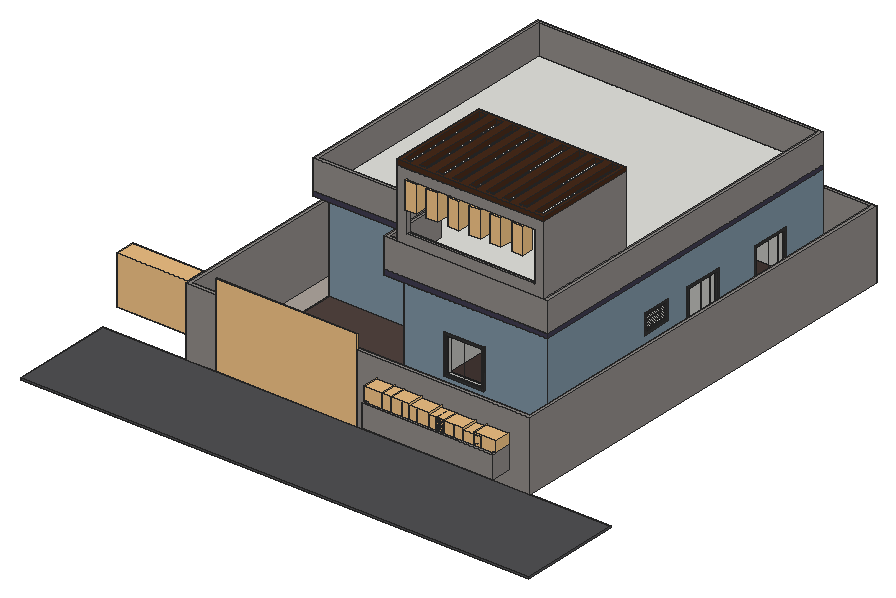
# SketchUp Ruby script. Lengths in inches.
U = 1.inch
M = Sketchup.active_model
def pt(a) = Geom::Point3d.new(a.map { |v| v * U })
def face(e, loops, mat)
  f = e.add_face(loops[0].map { |a| pt(a) })
  loops[1..].each { |l| e.add_face(l.map { |a| pt(a) }).erase! }
  f.material = f.back_material = mat if mat
  f
end
# faces: each face lists its corners as indices into pts; further lists are holes
def faces(e, pts, list, mat = nil) = list.each { |f| face(e, (f[0].is_a?(Array) ? f : [f]).map { |l| l.map { |i| pts[i] } }, mat) }
# xy, xz, yz: faces in a plane at the given z, y or x. An outline is a flat list of corners, or four numbers for a rectangle; further outlines are holes
def ring(l) = l.size == 4 ? [[l[0], l[1]], [l[2], l[1]], [l[2], l[3]], [l[0], l[3]]] : l.each_slice(2).to_a
def flat(e, list, mat, &to3) = list.each { |f| face(e, (f[0].is_a?(Array) ? f : [f]).map { |l| ring(l).map { |u, v| to3.(u, v) } }, mat) }
def xy(e, z, list, mat = nil) = flat(e, list, mat) { |x, y| [x, y, z] }
def xz(e, y, list, mat = nil) = flat(e, list, mat) { |x, z| [x, y, z] }
def yz(e, x, list, mat = nil) = flat(e, list, mat) { |y, z| [x, y, z] }
def lines(e, pts, list) = list.each { |a, b| e.add_line(pt(pts[a]), pt(pts[b])) }
# prism: a flat outline (further loops are holes) pulled along v
def prism(e, loops, v, mat = nil)
  f = face(e, loops, mat); d = Geom::Vector3d.new(v.map { |x| x * U })
  f.pushpull(f.normal.samedirection?(d) ? d.length : -d.length)
end
def box(e, o, s, mat = nil) = prism(e, [[o, [o[0] + s[0], o[1], o[2]], [o[0] + s[0], o[1] + s[1], o[2]], [o[0], o[1] + s[1], o[2]]]], [0, 0, s[2]], mat)
def at(x, y, z, deg = 0) = Geom::Transformation.translation(pt([x, y, z])) * Geom::Transformation.rotation(ORIGIN, Z_AXIS, deg.degrees)
def axes(o, x, y, z) = Geom::Transformation.new([*x, 0, *y, 0, *z, 0, *pt(o).to_a, 1])
def part(name) = M.definitions.add(name)
# library, detail: a bought-in or finely detailed component or shape, given as its bounding box
def library(name, o, s) = part(name).tap { |d| box(d.entities, o, s) }
def detail(e, o, s) = box(e.add_group.entities, o, s)
def put(e, d, t, mat = nil) = e.add_instance(d, t).tap { |i| i.material = mat if mat }
def group(e, t, mat = nil) = e.add_group.tap { |g| g.transformation = t; g.material = mat if mat }.entities
root = M.entities
M.materials.add("Asphalt A02 100cm").color = [81, 81, 83]
M.materials.add("Glass Green 001").color = [0, 0, 0]
M.materials["Glass Green 001"].alpha = 0.1
M.materials.add("Iron Blurry").color = [53, 53, 53]
M.materials.add("Marble Emperador Dark 150cm").color = [81, 67, 62]
M.materials.add("Tiles Simple H01 100cm").color = [173, 165, 157]
M.materials.add("Venetian Plaster Shadow 300cm").color = [61, 58, 77]
M.materials.add("Wall Paint Dusk Blue Semigloss 300cm").color = [122, 143, 157]
M.materials.add("Wall Paint Poised Taupe Semigloss 300cm").color = [140, 135, 132]
M.materials.add("Wenge Highgloss 300cm").color = [70, 42, 26]
c1 = library("gate 251k",[-0.18,0,0],[84.18,1.97,100.875])
c2 = library("Skimmia japonica Rubella 004",[-17.08,-16.64,-0.26],[33.2,34.59,28.81])
c3 = library("Hanging Plant 111-02",[-6.97,-7.06,-31.95],[13.94,14.12,31.95])
c4 = library("Dome Light",[-12,-12,0],[24,24,12])
c5 = part("Group\#31")
box(c5.entities,[0,0,0],[0.31,22,44])
c6 = part("Group\#33")
box(c6.entities,[0,0,0],[22,0.31,44])
c7 = part("Group\#35")
box(c7.entities,[0,0,0],[0.31,32,2])
c8 = part("Group\#37")
box(c8.entities,[-0.31,0,0],[0.31,22,44])
c9 = part("Group\#39")
box(c9.entities,[-0.31,0,0],[0.31,22,44])
c10 = part("Group\#41")
box(c10.entities,[0,0,0],[0.31,22,44])
c11 = part("Group\#43")
box(c11.entities,[0,0,0],[0.81,22,44])
c12 = part("Group\#45")
box(c12.entities,[0,0,0],[0.31,16,44])
put(root,c1,axes([309.25,125.79,8.27],[-2.04321,0,0],[0,1,0],[0,0,1]))
put(root,c2,axes([351.27,123.2,31.01],[1,0,0],[0,1,0],[0,0,1.35]))
put(root,c2,axes([373.16,123.2,31],[1,0,0],[0,1,0],[0,0,1.34812]))
put(root,c2,axes([397.15,123.2,30.99],[1,0,0],[0,1,0],[0,0,1.29341]))
put(root,c2,axes([415.51,123.2,30.98],[1,0,0],[0,1,0],[0,0,1.24092]))
put(root,c2,axes([439.16,123.2,30.97],[1,0,0],[0,1,0],[0,0,1.23466]))
put(root,c2,axes([461.16,123.2,30.96],[1,0,0],[0,1,0],[0,0,1.17781]))
put(root,c2,axes([482.18,123.2,30.98],[0.80733,0,0],[0,1,0],[0,0,1.24301]))
put(root,c3,at(320.25,202.29,248.27))
put(root,c3,at(345.8,202.29,248.27))
put(root,c3,at(372.54,202.29,248.27))
put(root,c3,at(398.6,202.29,248.27))
put(root,c3,at(423.8,202.29,248.27))
put(root,c3,at(450.02,202.29,248.27))
put(root,c4,axes([12.81,197.79,-6.4],[3.6267,0,0],[0,1,0],[0,0,4.8972]))
g1 = group(root,at(137.625,197.79,14.27))
xy(g1,0,[[0,0,172,0,172,101,136.6875,101,136.6875,105.5,172,105.5,172,138,181,138,181,9,339,9,339,133.5,217,133.5,217,196.5,227.5,196.5,227.5,192,221.5,192,221.5,138,264.5,138,264.5,143.4375,269,143.4375,269,138,339,138,339,192,269,192,269,179.4375,264.5,179.4375,264.5,192,263.5,192,263.5,196.5,339,196.5,339,274.5,224.5,274.5,224.5,279,339,279,339,411,176.5,411,176.5,279,188.5,279,188.5,274.5,160,274.5,160,279,172,279,172,411,9,411,9,279,124,279,124,274.5,85.5,274.5,85.5,202.5,81,202.5,81,274.5,9,274.5,9,154.5,81,154.5,81,166.5,85.5,166.5,85.5,150,9,150,9,105.5,81,105.5,81,114,85.5,114,85.5,105.5,100.6875,105.5,100.6875,101,0,101]],"Marble Emperador Dark 150cm")
xy(g1,36,[[222.5625,0,270.5625,9],[172,29.875,181,77.875],[0,110.375,9,146.375],[0,193.375,9,241.375],[339,210.875,348,258.875],
  [339,313.625,348,361.625],[0,327.125,9,375.125]])
xy(g1,60,[[339,145.8125,348,181.8125]])
xy(g1,84,[[222.5625,0,270.5625,9],[172,29.875,181,77.875],[100.6875,101,136.6875,105.5],[0,110.375,9,146.375],[81,114,85.5,150],
  [181,133.5,217,138],[264.5,143.4375,269,179.4375],[339,145.8125,348,181.8125],[81,166.5,85.5,202.5],[227.5,192,263.5,196.5],
  [0,193.375,9,241.375],[339,210.875,348,258.875],[124,274.5,160,279],[188.5,274.5,224.5,279],[339,313.625,348,361.625],
  [0,327.125,9,375.125]])
xy(g1,120,[[[172,0,348,0,348,420,0,420,0,101,172,101],[85.5,105.5,85.5,274.5,339,274.5,339,196.5,217,196.5,217,138,172,138,172,105.5],[9,279,172,411],[176.5,279,339,411],[181,9,339,133.5],[9,154.5,81,274.5],[269,138,339,192],[9,105.5,81,150],[221.5,138,264.5,192]]])
xz(g1,0,[[[172,0,348,120],[222.5625,36,270.5625,84]]],"Wall Paint Dusk Blue Semigloss 300cm")
xz(g1,9,[[[181,0,339,120],[222.5625,36,270.5625,84]]])
xz(g1,29.875,[[172,36,181,84]])
xz(g1,77.875,[[172,36,181,84]])
xz(g1,101,[[0,0,100.6875,0,100.6875,84,136.6875,84,136.6875,0,172,0,172,120,0,120]],"Wall Paint Dusk Blue Semigloss 300cm")
xz(g1,105.5,[[9,0,81,120],[85.5,0,85.5,120,172,120,172,0,136.6875,0,136.6875,84,100.6875,84,100.6875,0]])
xz(g1,110.375,[[0,36,9,84]])
xz(g1,114,[[81,0,85.5,84]])
xz(g1,133.5,[[217,0,339,0,339,120,181,120,181,84,217,84]])
xz(g1,138,[[172,0,172,120,217,120,217,84,181,84,181,0],[221.5,0,264.5,120],[269,0,339,120]])
xz(g1,143.4375,[[264.5,0,269,84]])
xz(g1,145.8125,[[339,60,348,84]])
xz(g1,146.375,[[0,36,9,84]])
xz(g1,150,[[9,0,85.5,0,85.5,84,81,84,81,120,9,120]])
xz(g1,154.5,[[9,0,81,120]])
xz(g1,166.5,[[81,0,85.5,84]])
xz(g1,179.4375,[[264.5,0,269,84]])
xz(g1,181.8125,[[339,60,348,84]])
xz(g1,192,[[221.5,0,227.5,0,227.5,84,263.5,84,263.5,0,264.5,0,264.5,120,221.5,120],[269,0,339,120]])
xz(g1,193.375,[[0,36,9,84]])
xz(g1,196.5,[[217,0,217,120,339,120,339,0,263.5,0,263.5,84,227.5,84,227.5,0]])
xz(g1,202.5,[[81,0,85.5,84]])
xz(g1,210.875,[[339,36,348,84]])
xz(g1,241.375,[[0,36,9,84]])
xz(g1,258.875,[[339,36,348,84]])
xz(g1,274.5,[[9,0,81,120],[85.5,0,124,0,124,84,160,84,160,0,188.5,0,188.5,84,224.5,84,224.5,0,339,0,339,120,85.5,120]])
xz(g1,279,[[9,0,9,120,172,120,172,0,160,0,160,84,124,84,124,0],[176.5,0,176.5,120,339,120,339,0,224.5,0,224.5,84,188.5,84,188.5,0]])
xz(g1,313.625,[[339,36,348,84]])
xz(g1,327.125,[[0,36,9,84]])
xz(g1,361.625,[[339,36,348,84]])
xz(g1,375.125,[[0,36,9,84]])
xz(g1,411,[[9,0,172,120],[176.5,0,339,120]])
xz(g1,420,[[0,0,348,120]],"Wall Paint Dusk Blue Semigloss 300cm")
yz(g1,0,[[[101,0,420,120],[193.375,36,241.375,84],[327.125,36,375.125,84],[110.375,36,146.375,84]]],"Wall Paint Dusk Blue Semigloss 300cm")
yz(g1,9,[[[105.5,0,150,120],[110.375,36,146.375,84]],[[154.5,0,274.5,120],[193.375,36,241.375,84]],[[279,0,411,120],[327.125,36,375.125,84]]])
yz(g1,81,[[105.5,0,105.5,120,150,120,150,84,114,84,114,0],[154.5,0,154.5,120,274.5,120,274.5,0,202.5,0,202.5,84,166.5,84,166.5,0]])
yz(g1,85.5,[[105.5,0,114,0,114,84,150,84,150,0,166.5,0,166.5,84,202.5,84,202.5,0,274.5,0,274.5,120,105.5,120]])
yz(g1,100.6875,[[101,0,105.5,84]])
yz(g1,124,[[274.5,0,279,84]])
yz(g1,136.6875,[[101,0,105.5,84]])
yz(g1,160,[[274.5,0,279,84]])
yz(g1,172,[[105.5,0,138,120],[279,0,411,120]])
yz(g1,172,[[[0,0,101,120],[29.875,36,77.875,84]]],"Wall Paint Dusk Blue Semigloss 300cm")
yz(g1,176.5,[[279,0,411,120]])
yz(g1,181,[[[9,0,138,0,138,84,133.5,84,133.5,120,9,120],[29.875,36,77.875,84]]])
yz(g1,188.5,[[274.5,0,279,84]])
yz(g1,217,[[133.5,0,133.5,84,138,84,138,120,196.5,120,196.5,0]])
yz(g1,221.5,[[138,0,192,120]])
yz(g1,222.5625,[[0,36,9,84]])
yz(g1,224.5,[[274.5,0,279,84]])
yz(g1,227.5,[[192,0,196.5,84]])
yz(g1,263.5,[[192,0,196.5,84]])
yz(g1,264.5,[[138,0,138,120,192,120,192,0,179.4375,0,179.4375,84,143.4375,84,143.4375,0]])
yz(g1,269,[[138,0,143.4375,0,143.4375,84,179.4375,84,179.4375,0,192,0,192,120,138,120]])
yz(g1,270.5625,[[0,36,9,84]])
yz(g1,339,[[9,0,133.5,120],[[138,0,192,120],[145.8125,60,181.8125,84]],[[196.5,0,274.5,120],[210.875,36,258.875,84]],[[279,0,411,120],[313.625,36,361.625,84]]])
yz(g1,348,[[[0,0,420,120],[313.625,36,361.625,84],[210.875,36,258.875,84],[145.8125,60,181.8125,84]]],"Wall Paint Dusk Blue Semigloss 300cm")
g2 = group(g1,at(124,274.5,0))
prism(g2,[[[36,0,0],[36,0,84],[0,0,84],[0,0,0]],[[34,0,82],[34,0,2],[2,0,2],[2,0,82]]],[0,2.5,0],"Iron Blurry")
g3 = group(g2,at(2,0,2))
xy(g3,0,[[0,0,32,0.71]])
xy(g3,80,[[0,0,32,0.71]])
xz(g3,0,[[0,0,32,80]],"Wenge Highgloss 300cm")
xz(g3,0.71,[[0,0,32,80]],"Wenge Highgloss 300cm")
yz(g3,0,[[0,0,0.71,80]])
yz(g3,32,[[0,0,0.71,80]])
g4 = group(g3,at(3.03,0,34.73),"Iron Blurry")
box(g4,[0,-0.5,0],[1.9375,0.5,7])
g5 = group(g1,at(188.5,274.5,0))
prism(g5,[[[36,0,0],[36,0,84],[0,0,84],[0,0,0]],[[34,0,2],[2,0,2],[2,0,82],[34,0,82]]],[0,2.5,0],"Iron Blurry")
g6 = group(g5,at(2,0,2))
box(g6,[0,0,0],[32,0.71,80],"Wenge Highgloss 300cm")
g7 = group(g6,at(3.5,0,38.76),"Iron Blurry")
box(g7,[0,-0.5,0],[1.25,0.5,6.6875])
g8 = group(g1,at(85.5,166.5,0))
prism(g8,[[[0,36,0],[0,36,84],[0,0,84],[0,0,0]],[[0,2,82],[0,34,82],[0,34,2],[0,2,2]]],[-2.5,0,0],"Iron Blurry")
g9 = group(g8,at(0,2,2))
box(g9,[-0.71,0,0],[0.71,32,80],"Wenge Highgloss 300cm")
g10 = group(g9,at(0,4.2,35.38),"Iron Blurry")
box(g10,[0,0,0],[0.5,2.125,10.0625])
g11 = group(g1,at(85.5,114,0))
prism(g11,[[[0,36,0],[0,36,84],[0,0,84],[0,0,0]],[[0,34,82],[0,34,2],[0,2,2],[0,2,82]]],[-2.5,0,0],"Iron Blurry")
g12 = group(g11,at(0,2,2))
box(g12,[-0.71,0,0],[0.71,32,80],"Wenge Highgloss 300cm")
g13 = group(g12,at(0,3.99,36.46),"Iron Blurry")
box(g13,[0,0,0],[0.5,1.6875,7.375],"Iron Blurry")
g14 = group(g1,at(181,138,0))
prism(g14,[[[0,0,0],[0,0,84],[36,0,84],[36,0,0]],[[2,0,82],[2,0,2],[34,0,2],[34,0,82]]],[0,-2.5,0],"Iron Blurry")
g15 = group(g14,at(2,0,2))
box(g15,[0,-0.71,0],[32,0.71,80],"Wenge Highgloss 300cm")
g16 = group(g15,at(28.34,0,39.96),"Iron Blurry")
box(g16,[-1.1875,0,0],[1.1875,0.5,6.8125],"Iron Blurry")
g17 = group(g1,at(264.5,143.4375,0))
xy(g17,0,[[0,0,2.5,36]])
xy(g17,2,[[0,2,2.5,34]])
xy(g17,82,[[0,2,2.5,34]])
xy(g17,84,[[0,0,2.5,36]])
xz(g17,0,[[0,0,2.5,84]])
xz(g17,2,[[0,2,2.5,82]])
xz(g17,34,[[0,2,2.5,82]])
xz(g17,36,[[0,0,2.5,84]])
yz(g17,0,[[[0,0,36,84],[2,2,34,82]]],"Iron Blurry")
yz(g17,2.5,[[[0,0,36,84],[2,2,34,82]]])
g18 = group(g17,at(0,2,2))
xy(g18,0,[[0,0,0.71,32]])
xy(g18,80,[[0,0,0.71,32]])
xz(g18,0,[[0,0,0.71,80]])
xz(g18,32,[[0,0,0.71,80]])
yz(g18,0,[[0,0,32,80]],"Wenge Highgloss 300cm")
yz(g18,0.71,[[0,0,32,80]],"Wenge Highgloss 300cm")
g19 = group(g18,at(0,27.54,34.45),"Iron Blurry")
box(g19,[-0.5,-1.375,0],[0.5,1.375,6])
g20 = group(g1,at(227.5,196.5,0))
prism(g20,[[[0,0,0],[0,0,84],[36,0,84],[36,0,0]],[[34,0,82],[2,0,82],[2,0,2],[34,0,2]]],[0,-2.5,0],"Iron Blurry")
g21 = group(g20,at(2,0,2))
box(g21,[0,-0.71,0],[32,0.71,80],"Wenge Highgloss 300cm")
g22 = group(g21,at(28.05,0,39.33),"Iron Blurry")
box(g22,[-1.375,0,0],[1.375,0.5,6.25])
g23 = group(g1,at(100.6875,101,0))
prism(g23,[[[36,0,0],[36,0,84],[0,0,84],[0,0,0]],[[34,0,2],[2,0,2],[2,0,82],[34,0,82]]],[0,2.5,0],"Iron Blurry")
g24 = group(g23,at(2,0,2))
box(g24,[0,0,0],[32,0.71,80],"Wenge Highgloss 300cm")
g25 = group(g24,at(4.23,0,37.9375),"Iron Blurry")
box(g25,[0,-0.5,0],[1.25,0.5,6.875],"Iron Blurry")
g26 = group(g1,at(172,29.875,36))
xy(g26,0,[[-1.5,0,1.5,48]],"Iron Blurry")
xy(g26,2,[[-1.5,2,1.5,46]],"Iron Blurry")
xy(g26,46,[[-1.5,2,1.5,46]],"Iron Blurry")
xy(g26,48,[[-1.5,0,1.5,48]],"Iron Blurry")
xz(g26,0,[[-1.5,0,1.5,48]],"Iron Blurry")
xz(g26,2,[[-1.5,2,1.5,46]],"Iron Blurry")
xz(g26,46,[[-1.5,2,1.5,46]],"Iron Blurry")
xz(g26,48,[[-1.5,0,1.5,48]],"Iron Blurry")
yz(g26,-1.5,[[[0,0,48,48],[2,2,46,46]]],"Iron Blurry")
yz(g26,1.5,[[[0,0,48,48],[2,2,46,46]]],"Iron Blurry")
put(g26,c5,at(0.3125,24,2),"Glass Green 001")
put(g26,c5,at(0,2,2),"Glass Green 001")
g27 = group(g1,at(222.5625,0,36))
xy(g27,0,[[0,-1.5,48,1.5]],"Iron Blurry")
xy(g27,2,[[2,-1.5,46,1.5]],"Iron Blurry")
xy(g27,46,[[2,-1.5,46,1.5]],"Iron Blurry")
xy(g27,48,[[0,-1.5,48,1.5]],"Iron Blurry")
xz(g27,-1.5,[[[0,0,48,48],[2,2,46,46]]],"Iron Blurry")
xz(g27,1.5,[[[0,0,48,48],[2,2,46,46]]],"Iron Blurry")
yz(g27,0,[[-1.5,0,1.5,48]],"Iron Blurry")
yz(g27,2,[[-1.5,2,1.5,46]],"Iron Blurry")
yz(g27,46,[[-1.5,2,1.5,46]],"Iron Blurry")
yz(g27,48,[[-1.5,0,1.5,48]],"Iron Blurry")
put(g27,c6,at(2,0.25,2),"Glass Green 001")
put(g27,c6,at(24,-0.06,2),"Glass Green 001")
g28 = group(g1,at(348,145.8125,60))
xy(g28,0,[[-1.5,0,1.5,36]],"Iron Blurry")
xy(g28,2,[[-1.5,2,1.5,34]],"Iron Blurry")
xy(g28,22,[[-1.5,2,1.5,34]],"Iron Blurry")
xy(g28,24,[[-1.5,0,1.5,36]],"Iron Blurry")
xz(g28,0,[[-1.5,0,1.5,24]],"Iron Blurry")
xz(g28,2,[[-1.5,2,1.5,22]],"Iron Blurry")
xz(g28,34,[[-1.5,2,1.5,22]],"Iron Blurry")
xz(g28,36,[[-1.5,0,1.5,24]],"Iron Blurry")
yz(g28,-1.5,[[[0,0,36,24],[2,2,34,22]]],"Iron Blurry")
yz(g28,1.5,[[[0,0,36,24],[2,2,34,22]]],"Iron Blurry")
put(g28,c7,at(1.5,2,20),"Glass Green 001")
put(g28,c7,at(1.5,2,17),"Glass Green 001")
put(g28,c7,at(1.5,2,14),"Glass Green 001")
put(g28,c7,at(1.5,2,11),"Glass Green 001")
put(g28,c7,at(1.5,2,8),"Glass Green 001")
put(g28,c7,at(1.5,2,5),"Glass Green 001")
put(g28,c7,at(1.5,2,2),"Glass Green 001")
g29 = group(g1,at(348,210.875,36))
xy(g29,0,[[-1.5,0,1.5,48]],"Iron Blurry")
xy(g29,2,[[-1.5,2,1.5,46]],"Iron Blurry")
xy(g29,46,[[-1.5,2,1.5,46]],"Iron Blurry")
xy(g29,48,[[-1.5,0,1.5,48]],"Iron Blurry")
xz(g29,0,[[-1.5,0,1.5,48]],"Iron Blurry")
xz(g29,2,[[-1.5,2,1.5,46]],"Iron Blurry")
xz(g29,46,[[-1.5,2,1.5,46]],"Iron Blurry")
xz(g29,48,[[-1.5,0,1.5,48]],"Iron Blurry")
yz(g29,-1.5,[[[0,0,48,48],[2,2,46,46]]],"Iron Blurry")
yz(g29,1.5,[[[0,0,48,48],[2,2,46,46]]],"Iron Blurry")
put(g29,c8,at(-0.4375,2,2),"Glass Green 001")
put(g29,c8,at(-0.12,24,2),"Glass Green 001")
g30 = group(g1,at(348,313.625,36))
xy(g30,0,[[-1.5,0,1.5,48]],"Iron Blurry")
xy(g30,2,[[-1.5,2,1.5,46]],"Iron Blurry")
xy(g30,46,[[-1.5,2,1.5,46]],"Iron Blurry")
xy(g30,48,[[-1.5,0,1.5,48]],"Iron Blurry")
xz(g30,0,[[-1.5,0,1.5,48]],"Iron Blurry")
xz(g30,2,[[-1.5,2,1.5,46]],"Iron Blurry")
xz(g30,46,[[-1.5,2,1.5,46]],"Iron Blurry")
xz(g30,48,[[-1.5,0,1.5,48]],"Iron Blurry")
yz(g30,-1.5,[[[0,0,48,48],[2,2,46,46]]],"Iron Blurry")
yz(g30,1.5,[[[0,0,48,48],[2,2,46,46]]],"Iron Blurry")
put(g30,c9,at(-0.625,2,2),"Glass Green 001")
put(g30,c9,at(-0.31,24,2),"Glass Green 001")
g31 = group(g1,at(0,327.125,36))
xy(g31,0,[[-1.5,0,1.5,48]],"Iron Blurry")
xy(g31,2,[[-1.5,2,1.5,46]],"Iron Blurry")
xy(g31,46,[[-1.5,2,1.5,46]],"Iron Blurry")
xy(g31,48,[[-1.5,0,1.5,48]],"Iron Blurry")
xz(g31,0,[[-1.5,0,1.5,48]],"Iron Blurry")
xz(g31,2,[[-1.5,2,1.5,46]],"Iron Blurry")
xz(g31,46,[[-1.5,2,1.5,46]],"Iron Blurry")
xz(g31,48,[[-1.5,0,1.5,48]],"Iron Blurry")
yz(g31,-1.5,[[[0,0,48,48],[2,2,46,46]]],"Iron Blurry")
yz(g31,1.5,[[[0,0,48,48],[2,2,46,46]]],"Iron Blurry")
put(g31,c10,at(0.3125,24,2),"Glass Green 001")
put(g31,c10,at(0,2,2),"Glass Green 001")
g32 = group(g1,at(0,193.375,36))
xy(g32,0,[[-1.5,0,1.5,48]],"Iron Blurry")
xy(g32,2,[[-1.5,2,1.5,46]],"Iron Blurry")
xy(g32,46,[[-1.5,2,1.5,46]],"Iron Blurry")
xy(g32,48,[[-1.5,0,1.5,48]],"Iron Blurry")
xz(g32,0,[[-1.5,0,1.5,48]],"Iron Blurry")
xz(g32,2,[[-1.5,2,1.5,46]],"Iron Blurry")
xz(g32,46,[[-1.5,2,1.5,46]],"Iron Blurry")
xz(g32,48,[[-1.5,0,1.5,48]],"Iron Blurry")
yz(g32,-1.5,[[[0,0,48,48],[2,2,46,46]]],"Iron Blurry")
yz(g32,1.5,[[[0,0,48,48],[2,2,46,46]]],"Iron Blurry")
put(g32,c11,at(0.25,24,2),"Glass Green 001")
put(g32,c11,at(-0.56,2,2),"Glass Green 001")
g33 = group(g1,at(0,110.375,36))
xy(g33,0,[[-1.5,0,1.5,36]],"Iron Blurry")
xy(g33,2,[[-1.5,2,1.5,34]],"Iron Blurry")
xy(g33,46,[[-1.5,2,1.5,34]],"Iron Blurry")
xy(g33,48,[[-1.5,0,1.5,36]],"Iron Blurry")
xz(g33,0,[[-1.5,0,1.5,48]],"Iron Blurry")
xz(g33,2,[[-1.5,2,1.5,46]],"Iron Blurry")
xz(g33,34,[[-1.5,2,1.5,46]],"Iron Blurry")
xz(g33,36,[[-1.5,0,1.5,48]],"Iron Blurry")
yz(g33,-1.5,[[[0,0,36,48],[2,2,34,46]]],"Iron Blurry")
yz(g33,1.5,[[[0,0,36,48],[2,2,34,46]]],"Iron Blurry")
put(g33,c12,at(-0.25,18,2),"Glass Green 001")
put(g33,c12,at(-0.56,2,2),"Glass Green 001")
g34 = group(root,at(137.625,197.79,134.27))
xy(g34,0,[[148,0,148,77,0,77,0,420,348,420,348,0]],"Venetian Plaster Shadow 300cm")
xy(g34,6,[[152.5,4.5,343.5,4.5,343.5,415.5,4.5,415.5,4.5,81.5,152.5,81.5]])
xz(g34,0,[[148,0,348,6]],"Venetian Plaster Shadow 300cm")
xz(g34,77,[[0,0,148,6]],"Venetian Plaster Shadow 300cm")
xz(g34,420,[[0,0,348,6]],"Venetian Plaster Shadow 300cm")
yz(g34,0,[[77,0,420,6]],"Venetian Plaster Shadow 300cm")
yz(g34,148,[[0,0,77,6]],"Venetian Plaster Shadow 300cm")
yz(g34,348,[[0,0,420,6]],"Venetian Plaster Shadow 300cm")
g35 = group(g34,at(0,0,6))
xy(g35,0,[[[148,0,148,77,0,77,0,420,348,420,348,0],[152.5,4.5,343.5,4.5,343.5,415.5,4.5,415.5,4.5,81.5,152.5,81.5]]])
xy(g35,36,[[148,0,163.5,0,163.5,4.5,152.5,4.5,152.5,81.5,4.5,81.5,4.5,415.5,343.5,415.5,343.5,0,348,0,348,420,0,420,0,77,148,77]],"Wall Paint Poised Taupe Semigloss 300cm")
xz(g35,0,[[148,0,348,36]],"Wall Paint Poised Taupe Semigloss 300cm")
xz(g35,4.5,[[152.5,0,343.5,36]],"Wall Paint Poised Taupe Semigloss 300cm")
xz(g35,77,[[0,0,148,36]],"Wall Paint Poised Taupe Semigloss 300cm")
xz(g35,81.5,[[4.5,0,152.5,36]],"Wall Paint Poised Taupe Semigloss 300cm")
xz(g35,415.5,[[4.5,0,343.5,36]],"Wall Paint Poised Taupe Semigloss 300cm")
xz(g35,420,[[0,0,348,36]],"Wall Paint Poised Taupe Semigloss 300cm")
yz(g35,0,[[77,0,420,36]],"Wall Paint Poised Taupe Semigloss 300cm")
yz(g35,4.5,[[81.5,0,415.5,36]],"Wall Paint Poised Taupe Semigloss 300cm")
yz(g35,148,[[0,0,77,36]],"Wall Paint Poised Taupe Semigloss 300cm")
yz(g35,152.5,[[4.5,0,81.5,36]],"Wall Paint Poised Taupe Semigloss 300cm")
yz(g35,343.5,[[4.5,0,415.5,36]],"Wall Paint Poised Taupe Semigloss 300cm")
yz(g35,348,[[0,0,420,36]],"Wall Paint Poised Taupe Semigloss 300cm")
g36 = group(g35,at(163.5,0,36))
box(g36,[0,119.9375,-36],[9,4.5625,120],"Wall Paint Poised Taupe Semigloss 300cm")
xy(g36,0,[[0,0,0,4.5,175.5,4.5,175.5,124.5,180,124.5,180,0]],"Wall Paint Poised Taupe Semigloss 300cm")
xy(g36,12,[[12,0,168,4.5]],"Wall Paint Poised Taupe Semigloss 300cm")
xy(g36,72,[[12,0,168,4.5]],"Wall Paint Poised Taupe Semigloss 300cm")
xy(g36,84,[[0,0,180,0,180,76.18,175.5,76.18,175.5,4.5,0,4.5],[175.5,76.18,180,124.5]],"Wall Paint Poised Taupe Semigloss 300cm")
xz(g36,0,[[[0,0,180,84],[12,12,168,72]]],"Wall Paint Poised Taupe Semigloss 300cm")
xz(g36,4.5,[[[0,0,175.5,84],[12,12,168,72]]],"Wall Paint Poised Taupe Semigloss 300cm")
xz(g36,124.5,[[175.5,0,180,84]],"Wall Paint Poised Taupe Semigloss 300cm")
yz(g36,0,[[0,0,4.5,84]],"Wall Paint Poised Taupe Semigloss 300cm")
yz(g36,12,[[0,12,4.5,72]],"Wall Paint Poised Taupe Semigloss 300cm")
yz(g36,168,[[0,12,4.5,72]],"Wall Paint Poised Taupe Semigloss 300cm")
yz(g36,175.5,[[4.5,0,124.5,84]],"Wall Paint Poised Taupe Semigloss 300cm")
yz(g36,180,[[0,0,124.5,84]],"Wall Paint Poised Taupe Semigloss 300cm")
g37 = group(g36,at(0,4.5,84),"Wenge Highgloss 300cm")
prism(g37,[[[0,120,0],[180,120,0],[180,-4.5,0],[0,-4.5,0]],[[13.5,115.5,0],[4.5,115.5,0],[4.5,0,0],[13.5,0,0]],[[33.75,115.5,0],[24.75,115.5,0],[24.75,0,0],[33.75,0,0]],[[54,115.5,0],[45,115.5,0],[45,0,0],[54,0,0]],[[74.25,115.5,0],[65.25,115.5,0],[65.25,0,0],[74.25,0,0]],[[94.5,115.5,0],[85.5,115.5,0],[85.5,0,0],[94.5,0,0]],[[114.75,115.5,0],[105.75,115.5,0],[105.75,0,0],[114.75,0,0]],[[135,115.5,0],[126,115.5,0],[126,0,0],[135,0,0]],[[155.25,115.5,0],[146.25,115.5,0],[146.25,0,0],[155.25,0,0]],[[175.5,115.5,0],[166.5,115.5,0],[166.5,0,0],[175.5,0,0]]],[0,0,6],"Wenge Highgloss 300cm")
g38 = group(root,at(137.625,197.79,8.27),"Marble Emperador Dark 150cm")
box(g38,[0,0,0],[348,420,6],"Marble Emperador Dark 150cm")
g39 = group(root,at(101.625,125.79,8.27))
xy(g39,0,[[36,0,208,0,208,4.5,415.5,4.5,415.5,523.5,4.5,523.5,4.5,4.5,36,4.5]],"Tiles Simple H01 100cm")
xy(g39,84,[[0,0,36,0,36,4.5,4.5,4.5,4.5,523.5,415.5,523.5,415.5,4.5,208,4.5,208,0,420,0,420,528,0,528]],"Wall Paint Poised Taupe Semigloss 300cm")
xz(g39,0,[[0,0,36,84],[208,0,420,84]],"Wall Paint Poised Taupe Semigloss 300cm")
xz(g39,4.5,[[4.5,0,36,84],[208,0,415.5,84]],"Wall Paint Poised Taupe Semigloss 300cm")
xz(g39,523.5,[[4.5,0,415.5,84]],"Wall Paint Poised Taupe Semigloss 300cm")
xz(g39,528,[[0,0,420,84]],"Wall Paint Poised Taupe Semigloss 300cm")
yz(g39,0,[[0,0,528,84]],"Wall Paint Poised Taupe Semigloss 300cm")
yz(g39,4.5,[[4.5,0,523.5,84]],"Wall Paint Poised Taupe Semigloss 300cm")
yz(g39,36,[[0,0,4.5,84]],"Wall Paint Poised Taupe Semigloss 300cm")
yz(g39,208,[[0,0,4.5,84]],"Wall Paint Poised Taupe Semigloss 300cm")
yz(g39,415.5,[[4.5,0,523.5,84]],"Wall Paint Poised Taupe Semigloss 300cm")
yz(g39,420,[[0,0,528,84]],"Wall Paint Poised Taupe Semigloss 300cm")
g40 = group(g39,at(234.2,0,18.01))
xy(g40,0,[[0,-24.3125,159.375,0]],"Wall Paint Poised Taupe Semigloss 300cm")
xy(g40,4.625,[[2.59,-21.72,156.78,-2.59]],"Wall Paint Poised Taupe Semigloss 300cm")
xy(g40,27.375,[[[0,-24.3125,159.375,0],[2.59,-21.72,156.78,-2.59]]],"Wall Paint Poised Taupe Semigloss 300cm")
xz(g40,-24.3125,[[0,0,159.375,27.375]],"Wall Paint Poised Taupe Semigloss 300cm")
xz(g40,-21.72,[[2.59,4.625,156.78,27.375]],"Wall Paint Poised Taupe Semigloss 300cm")
xz(g40,-2.59,[[2.59,4.625,156.78,27.375]],"Wall Paint Poised Taupe Semigloss 300cm")
xz(g40,0,[[0,0,159.375,27.375]],"Wall Paint Poised Taupe Semigloss 300cm")
yz(g40,0,[[-24.3125,0,0,27.375]],"Wall Paint Poised Taupe Semigloss 300cm")
yz(g40,2.59,[[-21.72,4.625,-2.59,27.375]],"Wall Paint Poised Taupe Semigloss 300cm")
yz(g40,156.78,[[-21.72,4.625,-2.59,27.375]],"Wall Paint Poised Taupe Semigloss 300cm")
yz(g40,159.375,[[-24.3125,0,0,27.375]],"Wall Paint Poised Taupe Semigloss 300cm")
g41 = group(root,at(101.625,0,8.27),"Asphalt A02 100cm")
box(g41,[-101.625,0,-2],[620.34,125.79,2],"Asphalt A02 100cm")
